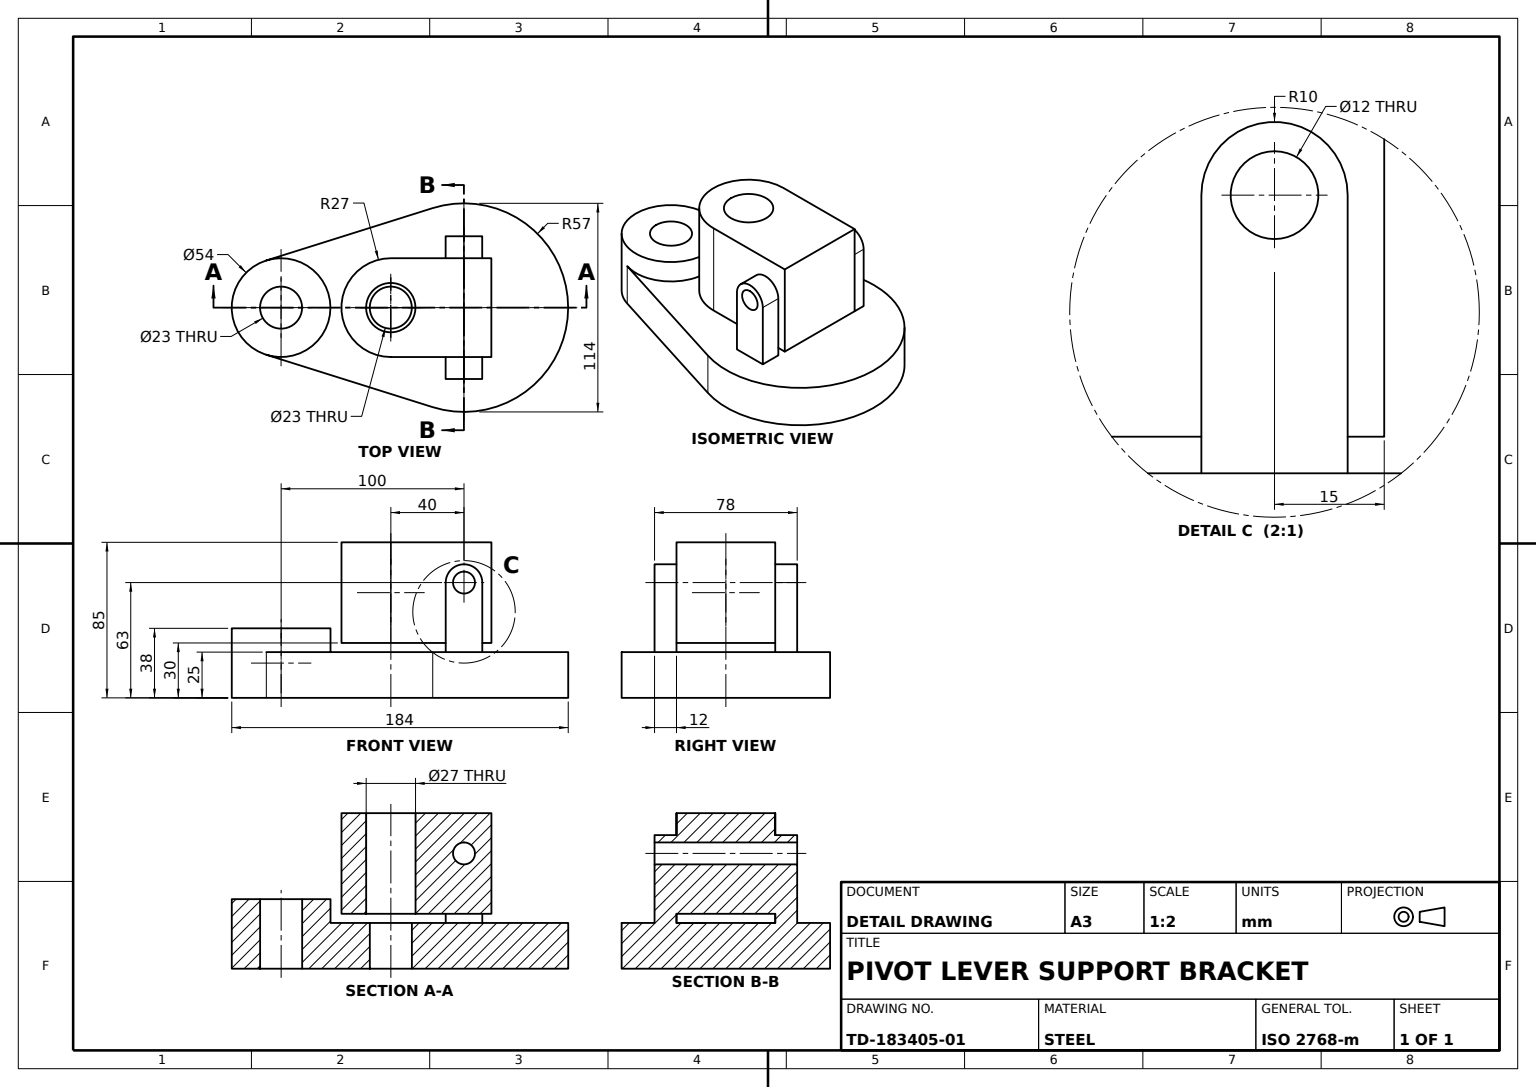
ISO-10303-21;
HEADER;
FILE_DESCRIPTION((''),'2;1');
FILE_NAME('','',(''),(''),'','','');
FILE_SCHEMA(('AUTOMOTIVE_DESIGN'));
ENDSEC;
DATA;
#1=APPLICATION_CONTEXT('');
#2=PRODUCT_CONTEXT('',#1,'mechanical');
#3=PRODUCT('','','',(#2));
#4=PRODUCT_DEFINITION_FORMATION('','',#3);
#5=PRODUCT_DEFINITION_CONTEXT('',#1,'design');
#6=PRODUCT_DEFINITION('','',#4,#5);
#7=PRODUCT_DEFINITION_SHAPE('','',#6);
#8=(LENGTH_UNIT()NAMED_UNIT(*)SI_UNIT(.MILLI.,.METRE.));
#9=(NAMED_UNIT(*)PLANE_ANGLE_UNIT()SI_UNIT($,.RADIAN.));
#10=(NAMED_UNIT(*)SI_UNIT($,.STERADIAN.)SOLID_ANGLE_UNIT());
#11=UNCERTAINTY_MEASURE_WITH_UNIT(LENGTH_MEASURE(0.005),#8,'distance_accuracy_value','');
#12=(GEOMETRIC_REPRESENTATION_CONTEXT(3)GLOBAL_UNCERTAINTY_ASSIGNED_CONTEXT((#11))GLOBAL_UNIT_ASSIGNED_CONTEXT((#8,#9,#10))REPRESENTATION_CONTEXT('',''));
#13=CARTESIAN_POINT('',(15.,27.,30.));
#14=VERTEX_POINT('',#13);
#15=CARTESIAN_POINT('',(10.,27.,30.));
#16=VERTEX_POINT('',#15);
#17=DIRECTION('',(-1.,0.,0.));
#18=VECTOR('',#17,1000.);
#19=LINE('',#13,#18);
#20=EDGE_CURVE('',#14,#16,#19,.T.);
#21=ORIENTED_EDGE('',*,*,#20,.T.);
#22=CARTESIAN_POINT('',(10.,27.,63.));
#23=VERTEX_POINT('',#22);
#24=CARTESIAN_POINT('',(10.,27.,0.));
#25=DIRECTION('',(0.,0.,1.));
#26=VECTOR('',#25,1000.);
#27=LINE('',#24,#26);
#28=EDGE_CURVE('',#16,#23,#27,.T.);
#29=ORIENTED_EDGE('',*,*,#28,.T.);
#30=CARTESIAN_POINT('',(-10.,27.,63.));
#31=VERTEX_POINT('',#30);
#32=CARTESIAN_POINT('',(0.,27.,63.));
#33=DIRECTION('',(0.,-1.,0.));
#34=DIRECTION('',(1.,0.,0.));
#35=AXIS2_PLACEMENT_3D('',#32,#33,#34);
#36=CIRCLE('',#35,10.);
#37=EDGE_CURVE('',#23,#31,#36,.T.);
#38=ORIENTED_EDGE('',*,*,#37,.T.);
#39=CARTESIAN_POINT('',(-10.,27.,30.));
#40=VERTEX_POINT('',#39);
#41=DIRECTION('',(0.,0.,-1.));
#42=VECTOR('',#41,1000.);
#43=LINE('',#30,#42);
#44=EDGE_CURVE('',#31,#40,#43,.T.);
#45=ORIENTED_EDGE('',*,*,#44,.T.);
#46=CARTESIAN_POINT('',(-40.,27.,30.));
#47=VERTEX_POINT('',#46);
#48=EDGE_CURVE('',#40,#47,#19,.T.);
#49=ORIENTED_EDGE('',*,*,#48,.T.);
#50=CARTESIAN_POINT('',(-40.,27.,85.));
#51=VERTEX_POINT('',#50);
#52=LINE('',#50,#42);
#53=EDGE_CURVE('',#51,#47,#52,.T.);
#54=ORIENTED_EDGE('',*,*,#53,.F.);
#55=CARTESIAN_POINT('',(15.,27.,85.));
#56=VERTEX_POINT('',#55);
#57=LINE('',#55,#18);
#58=EDGE_CURVE('',#56,#51,#57,.T.);
#59=ORIENTED_EDGE('',*,*,#58,.F.);
#60=LINE('',#55,#42);
#61=EDGE_CURVE('',#56,#14,#60,.T.);
#62=ORIENTED_EDGE('',*,*,#61,.T.);
#63=EDGE_LOOP('',(#21,#29,#38,#45,#49,#54,#59,#62));
#64=FACE_BOUND('',#63,.T.);
#65=AXIS2_PLACEMENT_3D('',#55,#33,#41);
#66=PLANE('',#65);
#67=ADVANCED_FACE('',(#64),#66,.F.);
#68=CARTESIAN_POINT('',(-10.,-39.,63.));
#69=VERTEX_POINT('',#68);
#70=CARTESIAN_POINT('',(-10.,-27.,63.));
#71=VERTEX_POINT('',#70);
#72=DIRECTION('',(0.,1.,0.));
#73=VECTOR('',#72,1000.);
#74=LINE('',#68,#73);
#75=EDGE_CURVE('',#69,#71,#74,.T.);
#76=ORIENTED_EDGE('',*,*,#75,.T.);
#77=CARTESIAN_POINT('',(-10.,-27.,30.));
#78=VERTEX_POINT('',#77);
#79=LINE('',#70,#42);
#80=EDGE_CURVE('',#71,#78,#79,.T.);
#81=ORIENTED_EDGE('',*,*,#80,.T.);
#82=CARTESIAN_POINT('',(-10.,-27.,25.));
#83=VERTEX_POINT('',#82);
#84=EDGE_CURVE('',#78,#83,#79,.T.);
#85=ORIENTED_EDGE('',*,*,#84,.T.);
#86=CARTESIAN_POINT('',(-10.,-39.,25.));
#87=VERTEX_POINT('',#86);
#88=CARTESIAN_POINT('',(-10.,0.,25.));
#89=LINE('',#88,#73);
#90=EDGE_CURVE('',#87,#83,#89,.T.);
#91=ORIENTED_EDGE('',*,*,#90,.F.);
#92=LINE('',#68,#42);
#93=EDGE_CURVE('',#69,#87,#92,.T.);
#94=ORIENTED_EDGE('',*,*,#93,.F.);
#95=EDGE_LOOP('',(#76,#81,#85,#91,#94));
#96=FACE_BOUND('',#95,.T.);
#97=AXIS2_PLACEMENT_3D('',#68,#34,#41);
#98=PLANE('',#97);
#99=ADVANCED_FACE('',(#96),#98,.F.);
#100=CARTESIAN_POINT('',(0.,-39.,69.));
#101=VERTEX_POINT('',#100);
#102=CARTESIAN_POINT('',(0.,-39.,63.));
#103=AXIS2_PLACEMENT_3D('',#102,#72,#25);
#104=CIRCLE('',#103,6.);
#105=EDGE_CURVE('',#101,#101,#104,.T.);
#106=ORIENTED_EDGE('',*,*,#105,.T.);
#107=EDGE_LOOP('',(#106));
#108=FACE_BOUND('',#107,.T.);
#109=CARTESIAN_POINT('',(10.,-39.,63.));
#110=VERTEX_POINT('',#109);
#111=AXIS2_PLACEMENT_3D('',#102,#33,#34);
#112=CIRCLE('',#111,10.);
#113=EDGE_CURVE('',#110,#69,#112,.T.);
#114=ORIENTED_EDGE('',*,*,#113,.T.);
#115=ORIENTED_EDGE('',*,*,#93,.T.);
#116=CARTESIAN_POINT('',(10.,-39.,25.));
#117=VERTEX_POINT('',#116);
#118=CARTESIAN_POINT('',(0.,-39.,25.));
#119=VECTOR('',#34,1000.);
#120=LINE('',#118,#119);
#121=EDGE_CURVE('',#87,#117,#120,.T.);
#122=ORIENTED_EDGE('',*,*,#121,.T.);
#123=CARTESIAN_POINT('',(10.,-39.,0.));
#124=LINE('',#123,#26);
#125=EDGE_CURVE('',#117,#110,#124,.T.);
#126=ORIENTED_EDGE('',*,*,#125,.T.);
#127=EDGE_LOOP('',(#114,#115,#122,#126));
#128=FACE_BOUND('',#127,.T.);
#129=AXIS2_PLACEMENT_3D('',#102,#33,#41);
#130=PLANE('',#129);
#131=ADVANCED_FACE('',(#108,#128),#130,.T.);
#132=CARTESIAN_POINT('',(-108.1,-25.756358,0.));
#133=VERTEX_POINT('',#132);
#134=CARTESIAN_POINT('',(-17.1,-54.374534,0.));
#135=VERTEX_POINT('',#134);
#136=DIRECTION('',(0.953939201,-0.3,0.));
#137=VECTOR('',#136,1000.);
#138=LINE('',#132,#137);
#139=EDGE_CURVE('',#133,#135,#138,.T.);
#140=ORIENTED_EDGE('',*,*,#139,.F.);
#141=CARTESIAN_POINT('',(-108.1,25.756358,0.));
#142=VERTEX_POINT('',#141);
#143=CARTESIAN_POINT('',(-100.,0.,0.));
#144=AXIS2_PLACEMENT_3D('',#143,#25,#34);
#145=CIRCLE('',#144,27.);
#146=EDGE_CURVE('',#142,#133,#145,.T.);
#147=ORIENTED_EDGE('',*,*,#146,.F.);
#148=CARTESIAN_POINT('',(-17.1,54.374534,0.));
#149=VERTEX_POINT('',#148);
#150=DIRECTION('',(-0.953939201,-0.3,0.));
#151=VECTOR('',#150,1000.);
#152=LINE('',#148,#151);
#153=EDGE_CURVE('',#149,#142,#152,.T.);
#154=ORIENTED_EDGE('',*,*,#153,.F.);
#155=CARTESIAN_POINT('',(0.,0.,0.));
#156=AXIS2_PLACEMENT_3D('',#155,#25,#34);
#157=CIRCLE('',#156,57.);
#158=EDGE_CURVE('',#135,#149,#157,.T.);
#159=ORIENTED_EDGE('',*,*,#158,.F.);
#160=EDGE_LOOP('',(#140,#147,#154,#159));
#161=FACE_BOUND('',#160,.T.);
#162=CARTESIAN_POINT('',(-28.5,0.,0.));
#163=VERTEX_POINT('',#162);
#164=CARTESIAN_POINT('',(-40.,0.,0.));
#165=AXIS2_PLACEMENT_3D('',#164,#25,#34);
#166=CIRCLE('',#165,11.5);
#167=EDGE_CURVE('',#163,#163,#166,.T.);
#168=ORIENTED_EDGE('',*,*,#167,.T.);
#169=EDGE_LOOP('',(#168));
#170=FACE_BOUND('',#169,.T.);
#171=CARTESIAN_POINT('',(-88.5,0.,0.));
#172=VERTEX_POINT('',#171);
#173=CIRCLE('',#144,11.5);
#174=EDGE_CURVE('',#172,#172,#173,.T.);
#175=ORIENTED_EDGE('',*,*,#174,.T.);
#176=EDGE_LOOP('',(#175));
#177=FACE_BOUND('',#176,.T.);
#178=PLANE('',#156);
#179=ADVANCED_FACE('',(#161,#170,#177),#178,.F.);
#180=ORIENTED_EDGE('',*,*,#53,.T.);
#181=CARTESIAN_POINT('',(-40.,-27.,30.));
#182=VERTEX_POINT('',#181);
#183=CARTESIAN_POINT('',(-40.,0.,30.));
#184=AXIS2_PLACEMENT_3D('',#183,#25,#34);
#185=CIRCLE('',#184,27.);
#186=EDGE_CURVE('',#47,#182,#185,.T.);
#187=ORIENTED_EDGE('',*,*,#186,.T.);
#188=CARTESIAN_POINT('',(-40.,-27.,85.));
#189=VERTEX_POINT('',#188);
#190=LINE('',#188,#42);
#191=EDGE_CURVE('',#189,#182,#190,.T.);
#192=ORIENTED_EDGE('',*,*,#191,.F.);
#193=CARTESIAN_POINT('',(-40.,0.,85.));
#194=AXIS2_PLACEMENT_3D('',#193,#25,#34);
#195=CIRCLE('',#194,27.);
#196=EDGE_CURVE('',#51,#189,#195,.T.);
#197=ORIENTED_EDGE('',*,*,#196,.F.);
#198=EDGE_LOOP('',(#180,#187,#192,#197));
#199=FACE_BOUND('',#198,.T.);
#200=AXIS2_PLACEMENT_3D('',#193,#41,#17);
#201=CYLINDRICAL_SURFACE('',#200,27.);
#202=ADVANCED_FACE('',(#199),#201,.T.);
#203=ORIENTED_EDGE('',*,*,#75,.F.);
#204=ORIENTED_EDGE('',*,*,#113,.F.);
#205=CARTESIAN_POINT('',(10.,-27.,63.));
#206=VERTEX_POINT('',#205);
#207=LINE('',#109,#73);
#208=EDGE_CURVE('',#110,#206,#207,.T.);
#209=ORIENTED_EDGE('',*,*,#208,.T.);
#210=CARTESIAN_POINT('',(0.,-27.,63.));
#211=AXIS2_PLACEMENT_3D('',#210,#33,#34);
#212=CIRCLE('',#211,10.);
#213=EDGE_CURVE('',#206,#71,#212,.T.);
#214=ORIENTED_EDGE('',*,*,#213,.T.);
#215=EDGE_LOOP('',(#203,#204,#209,#214));
#216=FACE_BOUND('',#215,.T.);
#217=CYLINDRICAL_SURFACE('',#103,10.);
#218=ADVANCED_FACE('',(#216),#217,.T.);
#219=CARTESIAN_POINT('',(-17.1,54.374534,25.));
#220=VERTEX_POINT('',#219);
#221=LINE('',#219,#42);
#222=EDGE_CURVE('',#220,#149,#221,.T.);
#223=ORIENTED_EDGE('',*,*,#222,.F.);
#224=CARTESIAN_POINT('',(-17.1,-54.374534,25.));
#225=VERTEX_POINT('',#224);
#226=CARTESIAN_POINT('',(0.,0.,25.));
#227=AXIS2_PLACEMENT_3D('',#226,#25,#34);
#228=CIRCLE('',#227,57.);
#229=EDGE_CURVE('',#225,#220,#228,.T.);
#230=ORIENTED_EDGE('',*,*,#229,.F.);
#231=LINE('',#224,#42);
#232=EDGE_CURVE('',#225,#135,#231,.T.);
#233=ORIENTED_EDGE('',*,*,#232,.T.);
#234=ORIENTED_EDGE('',*,*,#158,.T.);
#235=EDGE_LOOP('',(#223,#230,#233,#234));
#236=FACE_BOUND('',#235,.T.);
#237=AXIS2_PLACEMENT_3D('',#226,#41,#17);
#238=CYLINDRICAL_SURFACE('',#237,57.);
#239=ADVANCED_FACE('',(#236),#238,.T.);
#240=CARTESIAN_POINT('',(10.,-27.,25.));
#241=VERTEX_POINT('',#240);
#242=CARTESIAN_POINT('',(0.,-27.,25.));
#243=LINE('',#242,#119);
#244=EDGE_CURVE('',#83,#241,#243,.T.);
#245=ORIENTED_EDGE('',*,*,#244,.F.);
#246=ORIENTED_EDGE('',*,*,#84,.F.);
#247=CARTESIAN_POINT('',(10.,-27.,30.));
#248=VERTEX_POINT('',#247);
#249=LINE('',#181,#119);
#250=EDGE_CURVE('',#78,#248,#249,.T.);
#251=ORIENTED_EDGE('',*,*,#250,.T.);
#252=CARTESIAN_POINT('',(10.,-27.,0.));
#253=LINE('',#252,#26);
#254=EDGE_CURVE('',#241,#248,#253,.T.);
#255=ORIENTED_EDGE('',*,*,#254,.F.);
#256=EDGE_LOOP('',(#245,#246,#251,#255));
#257=FACE_BOUND('',#256,.T.);
#258=AXIS2_PLACEMENT_3D('',#210,#33,#41);
#259=PLANE('',#258);
#260=ADVANCED_FACE('',(#257),#259,.F.);
#261=EDGE_CURVE('',#248,#206,#253,.T.);
#262=ORIENTED_EDGE('',*,*,#261,.T.);
#263=ORIENTED_EDGE('',*,*,#208,.F.);
#264=ORIENTED_EDGE('',*,*,#125,.F.);
#265=CARTESIAN_POINT('',(10.,0.,25.));
#266=VECTOR('',#33,1000.);
#267=LINE('',#265,#266);
#268=EDGE_CURVE('',#241,#117,#267,.T.);
#269=ORIENTED_EDGE('',*,*,#268,.F.);
#270=ORIENTED_EDGE('',*,*,#254,.T.);
#271=EDGE_LOOP('',(#262,#263,#264,#269,#270));
#272=FACE_BOUND('',#271,.T.);
#273=AXIS2_PLACEMENT_3D('',#123,#17,#25);
#274=PLANE('',#273);
#275=ADVANCED_FACE('',(#272),#274,.F.);
#276=CARTESIAN_POINT('',(-53.5,0.,85.));
#277=VERTEX_POINT('',#276);
#278=CIRCLE('',#200,13.5);
#279=EDGE_CURVE('',#277,#277,#278,.T.);
#280=ORIENTED_EDGE('',*,*,#279,.T.);
#281=EDGE_LOOP('',(#280));
#282=FACE_BOUND('',#281,.T.);
#283=CARTESIAN_POINT('',(15.,-27.,85.));
#284=VERTEX_POINT('',#283);
#285=LINE('',#283,#73);
#286=EDGE_CURVE('',#284,#56,#285,.T.);
#287=ORIENTED_EDGE('',*,*,#286,.T.);
#288=ORIENTED_EDGE('',*,*,#58,.T.);
#289=ORIENTED_EDGE('',*,*,#196,.T.);
#290=LINE('',#188,#119);
#291=EDGE_CURVE('',#189,#284,#290,.T.);
#292=ORIENTED_EDGE('',*,*,#291,.T.);
#293=EDGE_LOOP('',(#287,#288,#289,#292));
#294=FACE_BOUND('',#293,.T.);
#295=PLANE('',#194);
#296=ADVANCED_FACE('',(#282,#294),#295,.T.);
#297=CARTESIAN_POINT('',(-10.,39.,63.));
#298=VERTEX_POINT('',#297);
#299=CARTESIAN_POINT('',(-10.,39.,25.));
#300=VERTEX_POINT('',#299);
#301=LINE('',#297,#42);
#302=EDGE_CURVE('',#298,#300,#301,.T.);
#303=ORIENTED_EDGE('',*,*,#302,.T.);
#304=CARTESIAN_POINT('',(-10.,27.,25.));
#305=VERTEX_POINT('',#304);
#306=LINE('',#88,#266);
#307=EDGE_CURVE('',#300,#305,#306,.T.);
#308=ORIENTED_EDGE('',*,*,#307,.T.);
#309=EDGE_CURVE('',#40,#305,#43,.T.);
#310=ORIENTED_EDGE('',*,*,#309,.F.);
#311=ORIENTED_EDGE('',*,*,#44,.F.);
#312=LINE('',#297,#266);
#313=EDGE_CURVE('',#298,#31,#312,.T.);
#314=ORIENTED_EDGE('',*,*,#313,.F.);
#315=EDGE_LOOP('',(#303,#308,#310,#311,#314));
#316=FACE_BOUND('',#315,.T.);
#317=AXIS2_PLACEMENT_3D('',#297,#17,#25);
#318=PLANE('',#317);
#319=ADVANCED_FACE('',(#316),#318,.T.);
#320=ORIENTED_EDGE('',*,*,#139,.T.);
#321=ORIENTED_EDGE('',*,*,#232,.F.);
#322=CARTESIAN_POINT('',(-108.1,-25.756358,25.));
#323=VERTEX_POINT('',#322);
#324=LINE('',#322,#137);
#325=EDGE_CURVE('',#323,#225,#324,.T.);
#326=ORIENTED_EDGE('',*,*,#325,.F.);
#327=LINE('',#322,#42);
#328=EDGE_CURVE('',#323,#133,#327,.T.);
#329=ORIENTED_EDGE('',*,*,#328,.T.);
#330=EDGE_LOOP('',(#320,#321,#326,#329));
#331=FACE_BOUND('',#330,.T.);
#332=DIRECTION('',(0.3,0.953939201,0.));
#333=DIRECTION('',(-0.953939201,0.3,0.));
#334=AXIS2_PLACEMENT_3D('',#322,#332,#333);
#335=PLANE('',#334);
#336=ADVANCED_FACE('',(#331),#335,.F.);
#337=CARTESIAN_POINT('',(-28.5,0.,25.));
#338=VERTEX_POINT('',#337);
#339=CARTESIAN_POINT('',(-40.,0.,25.));
#340=AXIS2_PLACEMENT_3D('',#339,#25,#34);
#341=CIRCLE('',#340,11.5);
#342=EDGE_CURVE('',#338,#338,#341,.T.);
#343=ORIENTED_EDGE('',*,*,#342,.T.);
#344=EDGE_LOOP('',(#343));
#345=FACE_BOUND('',#344,.T.);
#346=ORIENTED_EDGE('',*,*,#167,.F.);
#347=EDGE_LOOP('',(#346));
#348=FACE_BOUND('',#347,.T.);
#349=CARTESIAN_POINT('',(-40.,0.,-85.30177));
#350=AXIS2_PLACEMENT_3D('',#349,#41,#17);
#351=CYLINDRICAL_SURFACE('',#350,11.5);
#352=ADVANCED_FACE('',(#345,#348),#351,.F.);
#353=ORIENTED_EDGE('',*,*,#313,.T.);
#354=ORIENTED_EDGE('',*,*,#37,.F.);
#355=CARTESIAN_POINT('',(10.,39.,63.));
#356=VERTEX_POINT('',#355);
#357=LINE('',#355,#266);
#358=EDGE_CURVE('',#356,#23,#357,.T.);
#359=ORIENTED_EDGE('',*,*,#358,.F.);
#360=CARTESIAN_POINT('',(0.,39.,63.));
#361=AXIS2_PLACEMENT_3D('',#360,#33,#34);
#362=CIRCLE('',#361,10.);
#363=EDGE_CURVE('',#356,#298,#362,.T.);
#364=ORIENTED_EDGE('',*,*,#363,.T.);
#365=EDGE_LOOP('',(#353,#354,#359,#364));
#366=FACE_BOUND('',#365,.T.);
#367=AXIS2_PLACEMENT_3D('',#360,#33,#41);
#368=CYLINDRICAL_SURFACE('',#367,10.);
#369=ADVANCED_FACE('',(#366),#368,.T.);
#370=EDGE_CURVE('',#16,#40,#19,.T.);
#371=ORIENTED_EDGE('',*,*,#370,.T.);
#372=ORIENTED_EDGE('',*,*,#309,.T.);
#373=CARTESIAN_POINT('',(10.,27.,25.));
#374=VERTEX_POINT('',#373);
#375=CARTESIAN_POINT('',(0.,27.,25.));
#376=LINE('',#375,#119);
#377=EDGE_CURVE('',#305,#374,#376,.T.);
#378=ORIENTED_EDGE('',*,*,#377,.T.);
#379=EDGE_CURVE('',#374,#16,#27,.T.);
#380=ORIENTED_EDGE('',*,*,#379,.T.);
#381=EDGE_LOOP('',(#371,#372,#378,#380));
#382=FACE_BOUND('',#381,.T.);
#383=AXIS2_PLACEMENT_3D('',#32,#33,#41);
#384=PLANE('',#383);
#385=ADVANCED_FACE('',(#382),#384,.T.);
#386=ORIENTED_EDGE('',*,*,#61,.F.);
#387=ORIENTED_EDGE('',*,*,#286,.F.);
#388=CARTESIAN_POINT('',(15.,-27.,30.));
#389=VERTEX_POINT('',#388);
#390=LINE('',#283,#42);
#391=EDGE_CURVE('',#284,#389,#390,.T.);
#392=ORIENTED_EDGE('',*,*,#391,.T.);
#393=LINE('',#388,#73);
#394=EDGE_CURVE('',#389,#14,#393,.T.);
#395=ORIENTED_EDGE('',*,*,#394,.T.);
#396=EDGE_LOOP('',(#386,#387,#392,#395));
#397=FACE_BOUND('',#396,.T.);
#398=AXIS2_PLACEMENT_3D('',#283,#17,#25);
#399=PLANE('',#398);
#400=ADVANCED_FACE('',(#397),#399,.F.);
#401=CARTESIAN_POINT('',(0.,39.,57.));
#402=VERTEX_POINT('',#401);
#403=CIRCLE('',#367,6.);
#404=EDGE_CURVE('',#402,#402,#403,.T.);
#405=ORIENTED_EDGE('',*,*,#404,.F.);
#406=EDGE_LOOP('',(#405));
#407=FACE_BOUND('',#406,.T.);
#408=ORIENTED_EDGE('',*,*,#105,.F.);
#409=EDGE_LOOP('',(#408));
#410=FACE_BOUND('',#409,.T.);
#411=CYLINDRICAL_SURFACE('',#103,6.);
#412=ADVANCED_FACE('',(#407,#410),#411,.F.);
#413=ORIENTED_EDGE('',*,*,#279,.F.);
#414=EDGE_LOOP('',(#413));
#415=FACE_BOUND('',#414,.T.);
#416=CARTESIAN_POINT('',(-53.5,0.,30.));
#417=VERTEX_POINT('',#416);
#418=AXIS2_PLACEMENT_3D('',#183,#41,#17);
#419=CIRCLE('',#418,13.5);
#420=EDGE_CURVE('',#417,#417,#419,.T.);
#421=ORIENTED_EDGE('',*,*,#420,.T.);
#422=EDGE_LOOP('',(#421));
#423=FACE_BOUND('',#422,.T.);
#424=CYLINDRICAL_SURFACE('',#200,13.5);
#425=ADVANCED_FACE('',(#415,#423),#424,.F.);
#426=CARTESIAN_POINT('',(-111.5,0.,38.));
#427=VERTEX_POINT('',#426);
#428=CARTESIAN_POINT('',(-100.,0.,38.));
#429=AXIS2_PLACEMENT_3D('',#428,#41,#17);
#430=CIRCLE('',#429,11.5);
#431=EDGE_CURVE('',#427,#427,#430,.T.);
#432=ORIENTED_EDGE('',*,*,#431,.F.);
#433=EDGE_LOOP('',(#432));
#434=FACE_BOUND('',#433,.T.);
#435=ORIENTED_EDGE('',*,*,#174,.F.);
#436=EDGE_LOOP('',(#435));
#437=FACE_BOUND('',#436,.T.);
#438=CYLINDRICAL_SURFACE('',#429,11.5);
#439=ADVANCED_FACE('',(#434,#437),#438,.F.);
#440=ORIENTED_EDGE('',*,*,#431,.T.);
#441=EDGE_LOOP('',(#440));
#442=FACE_BOUND('',#441,.T.);
#443=CARTESIAN_POINT('',(-73.,0.,38.));
#444=VERTEX_POINT('',#443);
#445=AXIS2_PLACEMENT_3D('',#428,#25,#34);
#446=CIRCLE('',#445,27.);
#447=EDGE_CURVE('',#444,#444,#446,.T.);
#448=ORIENTED_EDGE('',*,*,#447,.T.);
#449=EDGE_LOOP('',(#448));
#450=FACE_BOUND('',#449,.T.);
#451=PLANE('',#445);
#452=ADVANCED_FACE('',(#442,#450),#451,.T.);
#453=ORIENTED_EDGE('',*,*,#394,.F.);
#454=EDGE_CURVE('',#248,#389,#249,.T.);
#455=ORIENTED_EDGE('',*,*,#454,.F.);
#456=ORIENTED_EDGE('',*,*,#250,.F.);
#457=EDGE_CURVE('',#182,#78,#249,.T.);
#458=ORIENTED_EDGE('',*,*,#457,.F.);
#459=ORIENTED_EDGE('',*,*,#186,.F.);
#460=ORIENTED_EDGE('',*,*,#48,.F.);
#461=ORIENTED_EDGE('',*,*,#370,.F.);
#462=ORIENTED_EDGE('',*,*,#20,.F.);
#463=EDGE_LOOP('',(#453,#455,#456,#458,#459,#460,#461,#462));
#464=FACE_BOUND('',#463,.T.);
#465=ORIENTED_EDGE('',*,*,#420,.F.);
#466=EDGE_LOOP('',(#465));
#467=FACE_BOUND('',#466,.T.);
#468=PLANE('',#184);
#469=ADVANCED_FACE('',(#464,#467),#468,.F.);
#470=ORIENTED_EDGE('',*,*,#447,.F.);
#471=EDGE_LOOP('',(#470));
#472=FACE_BOUND('',#471,.T.);
#473=ORIENTED_EDGE('',*,*,#146,.T.);
#474=ORIENTED_EDGE('',*,*,#328,.F.);
#475=CARTESIAN_POINT('',(-108.1,25.756358,25.));
#476=VERTEX_POINT('',#475);
#477=CARTESIAN_POINT('',(-100.,0.,25.));
#478=AXIS2_PLACEMENT_3D('',#477,#25,#34);
#479=CIRCLE('',#478,27.);
#480=EDGE_CURVE('',#476,#323,#479,.F.);
#481=ORIENTED_EDGE('',*,*,#480,.F.);
#482=LINE('',#475,#42);
#483=EDGE_CURVE('',#476,#142,#482,.T.);
#484=ORIENTED_EDGE('',*,*,#483,.T.);
#485=EDGE_LOOP('',(#473,#474,#481,#484));
#486=FACE_BOUND('',#485,.T.);
#487=AXIS2_PLACEMENT_3D('',#477,#41,#17);
#488=CYLINDRICAL_SURFACE('',#487,27.);
#489=ADVANCED_FACE('',(#472,#486),#488,.T.);
#490=LINE('',#219,#151);
#491=EDGE_CURVE('',#220,#476,#490,.T.);
#492=ORIENTED_EDGE('',*,*,#491,.T.);
#493=ORIENTED_EDGE('',*,*,#480,.T.);
#494=ORIENTED_EDGE('',*,*,#325,.T.);
#495=ORIENTED_EDGE('',*,*,#229,.T.);
#496=EDGE_LOOP('',(#492,#493,#494,#495));
#497=FACE_BOUND('',#496,.T.);
#498=ORIENTED_EDGE('',*,*,#342,.F.);
#499=EDGE_LOOP('',(#498));
#500=FACE_BOUND('',#499,.T.);
#501=CARTESIAN_POINT('',(10.,39.,25.));
#502=VERTEX_POINT('',#501);
#503=CARTESIAN_POINT('',(0.,39.,25.));
#504=LINE('',#503,#119);
#505=EDGE_CURVE('',#300,#502,#504,.T.);
#506=ORIENTED_EDGE('',*,*,#505,.T.);
#507=LINE('',#265,#73);
#508=EDGE_CURVE('',#374,#502,#507,.T.);
#509=ORIENTED_EDGE('',*,*,#508,.F.);
#510=ORIENTED_EDGE('',*,*,#377,.F.);
#511=ORIENTED_EDGE('',*,*,#307,.F.);
#512=EDGE_LOOP('',(#506,#509,#510,#511));
#513=FACE_BOUND('',#512,.T.);
#514=ORIENTED_EDGE('',*,*,#244,.T.);
#515=ORIENTED_EDGE('',*,*,#268,.T.);
#516=ORIENTED_EDGE('',*,*,#121,.F.);
#517=ORIENTED_EDGE('',*,*,#90,.T.);
#518=EDGE_LOOP('',(#514,#515,#516,#517));
#519=FACE_BOUND('',#518,.T.);
#520=PLANE('',#227);
#521=ADVANCED_FACE('',(#497,#500,#513,#519),#520,.T.);
#522=ORIENTED_EDGE('',*,*,#404,.T.);
#523=EDGE_LOOP('',(#522));
#524=FACE_BOUND('',#523,.T.);
#525=ORIENTED_EDGE('',*,*,#363,.F.);
#526=CARTESIAN_POINT('',(10.,39.,0.));
#527=LINE('',#526,#26);
#528=EDGE_CURVE('',#502,#356,#527,.T.);
#529=ORIENTED_EDGE('',*,*,#528,.F.);
#530=ORIENTED_EDGE('',*,*,#505,.F.);
#531=ORIENTED_EDGE('',*,*,#302,.F.);
#532=EDGE_LOOP('',(#525,#529,#530,#531));
#533=FACE_BOUND('',#532,.T.);
#534=PLANE('',#367);
#535=ADVANCED_FACE('',(#524,#533),#534,.F.);
#536=ORIENTED_EDGE('',*,*,#222,.T.);
#537=ORIENTED_EDGE('',*,*,#153,.T.);
#538=ORIENTED_EDGE('',*,*,#483,.F.);
#539=ORIENTED_EDGE('',*,*,#491,.F.);
#540=EDGE_LOOP('',(#536,#537,#538,#539));
#541=FACE_BOUND('',#540,.T.);
#542=DIRECTION('',(0.3,-0.953939201,0.));
#543=DIRECTION('',(0.953939201,0.3,0.));
#544=AXIS2_PLACEMENT_3D('',#219,#542,#543);
#545=PLANE('',#544);
#546=ADVANCED_FACE('',(#541),#545,.F.);
#547=ORIENTED_EDGE('',*,*,#28,.F.);
#548=ORIENTED_EDGE('',*,*,#379,.F.);
#549=ORIENTED_EDGE('',*,*,#508,.T.);
#550=ORIENTED_EDGE('',*,*,#528,.T.);
#551=ORIENTED_EDGE('',*,*,#358,.T.);
#552=EDGE_LOOP('',(#547,#548,#549,#550,#551));
#553=FACE_BOUND('',#552,.T.);
#554=AXIS2_PLACEMENT_3D('',#526,#34,#41);
#555=PLANE('',#554);
#556=ADVANCED_FACE('',(#553),#555,.T.);
#557=ORIENTED_EDGE('',*,*,#457,.T.);
#558=ORIENTED_EDGE('',*,*,#80,.F.);
#559=ORIENTED_EDGE('',*,*,#213,.F.);
#560=ORIENTED_EDGE('',*,*,#261,.F.);
#561=ORIENTED_EDGE('',*,*,#454,.T.);
#562=ORIENTED_EDGE('',*,*,#391,.F.);
#563=ORIENTED_EDGE('',*,*,#291,.F.);
#564=ORIENTED_EDGE('',*,*,#191,.T.);
#565=EDGE_LOOP('',(#557,#558,#559,#560,#561,#562,#563,#564));
#566=FACE_BOUND('',#565,.T.);
#567=AXIS2_PLACEMENT_3D('',#188,#72,#25);
#568=PLANE('',#567);
#569=ADVANCED_FACE('',(#566),#568,.F.);
#570=CLOSED_SHELL('',(#67,#99,#131,#179,#202,#218,#239,#260,#275,#296,#319,#336,#352,#369,#385,#400,#412,#425,#439,#452,#469,#489,#521,#535,#546,#556,#569));
#571=MANIFOLD_SOLID_BREP('',#570);
#572=ADVANCED_BREP_SHAPE_REPRESENTATION('',(#571),#12);
#573=SHAPE_DEFINITION_REPRESENTATION(#7,#572);
ENDSEC;
END-ISO-10303-21;
